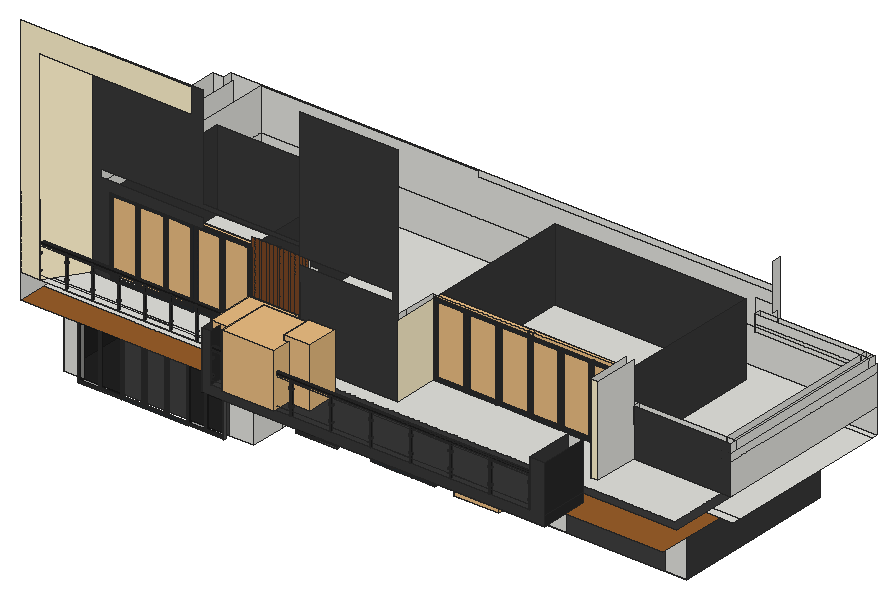
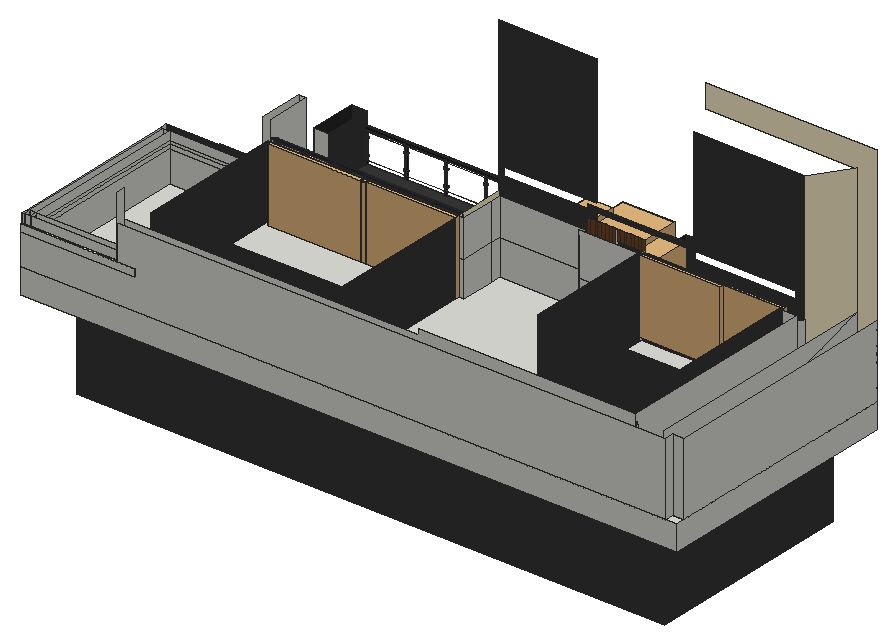
# SketchUp Ruby script. Lengths in inches.
U = 1.inch
M = Sketchup.active_model
def pt(a) = Geom::Point3d.new(a.map { |v| v * U })
def face(e, loops, mat)
  f = e.add_face(loops[0].map { |a| pt(a) })
  loops[1..].each { |l| e.add_face(l.map { |a| pt(a) }).erase! }
  f.material = f.back_material = mat if mat
  f
end
# faces: each face lists its corners as indices into pts; further lists are holes
def faces(e, pts, list, mat = nil) = list.each { |f| face(e, (f[0].is_a?(Array) ? f : [f]).map { |l| l.map { |i| pts[i] } }, mat) }
# xy, xz, yz: faces in a plane at the given z, y or x. An outline is a flat list of corners, or four numbers for a rectangle; further outlines are holes
def ring(l) = l.size == 4 ? [[l[0], l[1]], [l[2], l[1]], [l[2], l[3]], [l[0], l[3]]] : l.each_slice(2).to_a
def flat(e, list, mat, &to3) = list.each { |f| face(e, (f[0].is_a?(Array) ? f : [f]).map { |l| ring(l).map { |u, v| to3.(u, v) } }, mat) }
def xy(e, z, list, mat = nil) = flat(e, list, mat) { |x, y| [x, y, z] }
def xz(e, y, list, mat = nil) = flat(e, list, mat) { |x, z| [x, y, z] }
def yz(e, x, list, mat = nil) = flat(e, list, mat) { |y, z| [x, y, z] }
def lines(e, pts, list) = list.each { |a, b| e.add_line(pt(pts[a]), pt(pts[b])) }
# prism: a flat outline (further loops are holes) pulled along v
def prism(e, loops, v, mat = nil)
  f = face(e, loops, mat); d = Geom::Vector3d.new(v.map { |x| x * U })
  f.pushpull(f.normal.samedirection?(d) ? d.length : -d.length)
end
def box(e, o, s, mat = nil) = prism(e, [[o, [o[0] + s[0], o[1], o[2]], [o[0] + s[0], o[1] + s[1], o[2]], [o[0], o[1] + s[1], o[2]]]], [0, 0, s[2]], mat)
def at(x, y, z, deg = 0) = Geom::Transformation.translation(pt([x, y, z])) * Geom::Transformation.rotation(ORIGIN, Z_AXIS, deg.degrees)
def axes(o, x, y, z) = Geom::Transformation.new([*x, 0, *y, 0, *z, 0, *pt(o).to_a, 1])
def part(name) = M.definitions.add(name)
# library, detail: a bought-in or finely detailed component or shape, given as its bounding box
def library(name, o, s) = part(name).tap { |d| box(d.entities, o, s) }
def detail(e, o, s) = box(e.add_group.entities, o, s)
def put(e, d, t, mat = nil) = e.add_instance(d, t).tap { |i| i.material = mat if mat }
def group(e, t, mat = nil) = e.add_group.tap { |g| g.transformation = t; g.material = mat if mat }.entities
root = M.entities
M.materials.add("Glass_Tinted_Gray").color = [0, 0, 0]
M.materials["Glass_Tinted_Gray"].alpha = 0.125
M.materials.add("Wine2").color = [0, 0, 0]
M.materials["Wine2"].alpha = 0
M.materials.add("[0130_Gainsboro]").color = [39, 45, 50]
M.materials.add("[0131_Silver]").color = [28, 28, 28]
M.materials.add("[0135_DarkGray]").color = [81, 81, 81]
M.materials.add("[Color D01]").color = [255, 242, 204]
M.materials.add("[Color M08]").color = [56, 56, 56]
M.materials.add("[Granite Dark Gray]").color = [40, 40, 40]
M.materials.add("[Mirror 02]").color = [229, 229, 229]
M.materials.add("[Terrazzo Light Blue]").color = [196, 214, 227]
M.materials.add("[Translucent_Glass_Blue]").color = [255, 255, 255]
M.materials["[Translucent_Glass_Blue]"].alpha = 0
M.materials.add("[Wood Floor Dark]").color = [153, 94, 42]
M.materials.add("[Wood Veneer 01]").color = [120, 70, 37]
c1 = part("PENTEK_RP Fineline 50S_Sliding_DoorCase_E1")
box(c1.entities,[0,0,0],[1.51,3.66,99.27],"[0135_DarkGray]")
c2 = part("PENTEK_RP Fineline 50S_SlidingDooe_Case_E2")
box(c2.entities,[0,0,0],[96.25,3.66,1.51],"[0135_DarkGray]")
c3 = part("pentek_RP Fineline 50S_SlidingDoor_Case")
put(c3.entities,c1,at(97.76,0,0))
put(c3.entities,c2,at(1.51,0,0))
put(c3.entities,c1,at(0,0,0))
put(c3.entities,c2,at(1.51,0,97.76))
c4 = part("PENTEK_RP Fineline 50S_SlidingDoor_GlazingBead_2")
box(c4.entities,[0,0,0],[0.56,0.59,94.39],"[0135_DarkGray]")
c5 = part("PENTEK_RP Fineline 50S_SlidingDoor_Glass")
box(c5.entities,[0,0,0],[46.58,0.16,94.39],"Glass_Tinted_Gray")
c6 = part("PENTEK_RP Fineline 50S_SlidingDoor_GlazingBead")
box(c6.entities,[0,0,0],[45.47,0.59,0.56],"[0135_DarkGray]")
c7 = part("PENTEK_RP Fineline 50S_SlidingDoor_Leaf_E1")
xy(c7.entities,0,[[0,0,0.93,1.97],[0.93,1.57,1.49,1.97]],"[0135_DarkGray]")
xy(c7.entities,96.25,[[0,0,0.93,0,0.93,1.57,1.49,1.57,1.49,1.97,0,1.97]],"[0135_DarkGray]")
xz(c7.entities,0,[[0,0,0.93,96.25]],"[0135_DarkGray]")
xz(c7.entities,1.57,[[0.93,0,1.49,95.32],[0.93,95.32,1.49,96.25]],"[0135_DarkGray]")
xz(c7.entities,1.97,[[0,0,1.49,96.25]],"[0135_DarkGray]")
yz(c7.entities,0,[[0,0,1.97,96.25]],"[0135_DarkGray]")
yz(c7.entities,0.93,[[0,0,1.57,0.93],[0,0.93,1.57,95.32],[0,95.32,1.57,96.25]],"[0135_DarkGray]")
yz(c7.entities,1.49,[[1.57,0,1.97,95.32],[1.57,95.32,1.97,96.25]],"[0135_DarkGray]")
c8 = part("PENTEK_RP Fineline 50S_SlidingDoor_Leaf_E2")
xy(c8.entities,0,[[0,0,0,1.57,0.56,1.57,0.56,1.97,46.02,1.97,46.02,1.57,46.58,1.57,46.58,0]],"[0135_DarkGray]")
xy(c8.entities,0.93,[[0,0,46.58,1.57]],"[0135_DarkGray]")
xy(c8.entities,1.49,[[0.56,1.57,46.02,1.97]],"[0135_DarkGray]")
xz(c8.entities,0,[[0,0,46.58,0.93]],"[0135_DarkGray]")
xz(c8.entities,1.57,[[0,0,0.56,0.93],[46.02,0,46.58,0.93],[0.56,0.93,46.02,1.49]],"[0135_DarkGray]")
xz(c8.entities,1.97,[[0.56,0,46.02,1.49]],"[0135_DarkGray]")
yz(c8.entities,0,[[0,0,1.57,0.93]],"[0135_DarkGray]")
yz(c8.entities,0.56,[[1.57,0,1.97,0.93],[1.57,0.93,1.97,1.49]],"[0135_DarkGray]")
yz(c8.entities,46.02,[[1.57,0,1.97,0.93],[1.57,0.93,1.97,1.49]],"[0135_DarkGray]")
yz(c8.entities,46.58,[[0,0,1.57,0.93]],"[0135_DarkGray]")
c9 = part("PENTEK_RP Fineline S_SlidingDoor_Leaf1")
put(c9.entities,c4,at(0.93,0,0.93))
put(c9.entities,c4,at(46.96,0,0.93))
put(c9.entities,c5,at(1.49,1.42,0.93))
put(c9.entities,c6,at(1.49,0,0.93))
put(c9.entities,c5,at(1.49,0.59,0.93),"[Terrazzo Light Blue]")
put(c9.entities,c7,at(0,0,0))
put(c9.entities,c7,axes([48.44,0,0],[-1,0,0],[0,1,0],[0,0,1]))
put(c9.entities,c8,axes([0.93,0,96.25],[1,0,0],[0,1,0],[0,0,-1]))
put(c9.entities,c8,at(0.93,0,0))
put(c9.entities,c6,at(1.49,0,94.77))
c10 = part("PENTEK_RP Fineline 50S_SlidingDoor_Leaf2")
put(c10.entities,c5,at(1.49,1.42,0.93))
put(c10.entities,c6,at(1.49,0,94.77))
put(c10.entities,c4,at(46.96,0,0.93))
put(c10.entities,c5,at(1.49,0.59,0.93),"[Mirror 02]")
put(c10.entities,c4,at(0.93,0,0.93))
put(c10.entities,c7,at(0,0,0))
put(c10.entities,c7,axes([48.44,0,0],[-1,0,0],[0,1,0],[0,0,1]))
put(c10.entities,c6,at(1.49,0,0.93))
put(c10.entities,c8,axes([0.93,0,96.25],[1,0,0],[0,1,0],[0,0,-1]))
put(c10.entities,c8,at(0.93,0,0))
c11 = part("PENTEK - Slimmest Steel Sliding Door / Window\#1")
put(c11.entities,c3,at(0,-1.88,-0.09))
put(c11.entities,c9,at(1.51,-2.27,1.42))
put(c11.entities,c10,at(49.32,-0.3,1.42))
c12 = part("Framed glazing panel")
xy(c12.entities,0,[[0,-0.98,43.07,0],[0,0,43.07,1.4]],"[0130_Gainsboro]")
xy(c12.entities,0.3,[[0.3,-1.43,42.77,-0.98]],"[0130_Gainsboro]")
xy(c12.entities,2.95,[[2.95,-1.43,40.12,-0.63],[2.95,-0.63,40.12,0],[2.95,0,40.12,0.64],[2.95,0.64,40.12,1.4]],"[0130_Gainsboro]")
xy(c12.entities,3.54,[[3.54,-0.63,39.53,0],[3.54,0,39.53,0.64]],"[0130_Gainsboro]")
xy(c12.entities,111.8125,[[3.54,-0.63,39.53,0],[3.54,0,39.53,0.64]],"[0130_Gainsboro]")
xy(c12.entities,112.4,[[2.95,-1.43,40.12,-0.63],[2.95,-0.63,40.12,0],[2.95,0,40.12,0.64],[2.95,0.64,40.12,1.4]],"[0130_Gainsboro]")
xy(c12.entities,115.05,[[0.3,-1.43,42.77,-0.98]],"[0130_Gainsboro]")
xy(c12.entities,115.35,[[0,-0.98,43.07,0],[0,0,43.07,1.4]],"[0130_Gainsboro]")
xz(c12.entities,-1.43,[[[0.3,0.3,42.77,115.05],[2.95,2.95,40.12,112.4]]],"[0130_Gainsboro]")
xz(c12.entities,-0.98,[[[0,0,43.07,115.35],[0.3,0.3,42.77,115.05]]],"[0130_Gainsboro]")
xz(c12.entities,-0.63,[[[2.95,2.95,40.12,112.4],[3.54,3.54,39.53,111.8125]]],"[0130_Gainsboro]")
xz(c12.entities,0,[[3.54,3.54,39.53,111.8125]],"Wine2")
xz(c12.entities,0,[[[0,0,43.07,115.35],[2.95,2.95,40.12,112.4]],[[2.95,2.95,40.12,112.4],[3.54,3.54,39.53,111.8125]]],"[0130_Gainsboro]")
xz(c12.entities,0.64,[[[2.95,2.95,40.12,112.4],[3.54,3.54,39.53,111.8125]]],"[0130_Gainsboro]")
xz(c12.entities,1.4,[[[0,0,43.07,115.35],[2.95,2.95,40.12,112.4]]],"[0130_Gainsboro]")
yz(c12.entities,0,[[-0.98,0,0,115.35],[0,0,1.4,115.35]],"[0130_Gainsboro]")
yz(c12.entities,0.3,[[-1.43,0.3,-0.98,115.05]],"[0130_Gainsboro]")
yz(c12.entities,2.95,[[-1.43,2.95,-0.63,112.4],[-0.63,2.95,0,112.4],[0,2.95,0.64,112.4],[0.64,2.95,1.4,112.4]],"[0130_Gainsboro]")
yz(c12.entities,3.54,[[-0.63,3.54,0,111.8125],[0,3.54,0.64,111.8125]],"[0130_Gainsboro]")
yz(c12.entities,39.53,[[-0.63,3.54,0,111.8125],[0,3.54,0.64,111.8125]],"[0130_Gainsboro]")
yz(c12.entities,40.12,[[-1.43,2.95,-0.63,112.4],[-0.63,2.95,0,112.4],[0,2.95,0.64,112.4],[0.64,2.95,1.4,112.4]],"[0130_Gainsboro]")
yz(c12.entities,42.77,[[-1.43,0.3,-0.98,115.05]],"[0130_Gainsboro]")
yz(c12.entities,43.07,[[-0.98,0,0,115.35],[0,0,1.4,115.35]],"[0130_Gainsboro]")
c13 = part("Glazed screen")
put(c13.entities,c12,axes([90.57,1.43,0],[1.05148,0,0],[0,1,0],[0,0,1]))
put(c13.entities,c12,axes([0,1.43,0],[1.05148,0,0],[0,1,0],[0,0,1]))
put(c13.entities,c12,axes([45.29,1.43,0],[1.05148,0,0],[0,1,0],[0,0,1]))
c14 = library("元件\#5",[-4.39,0,0],[5.37,35.83,90.55])
c15 = library("Group5_1",[-7.56,-66.38,0.11],[6.33,135.04,120.95])
c16 = library("Pot+Plant",[-20.81,-17.08,-0.03],[39.86,39.43,41.33])
c17 = library("Potted broadleaf plant",[-29.7,0,-10.87],[31.67,38.52,72.45])
c18 = library("Plant+++Pot",[-21.48,-119.36,-205.6875],[86.44,86.43,89.41])
c19 = part("Monstera_Pot_Quarter")
detail(c19.entities,[0.23,0.23,0],[9.32,9.32,13.9])
c20 = part("Monstera_Stem")
p = [[0.53,2.46,1.55],[0.55,2.41,0.71],[0.58,2.34,0.01],[0.58,2.59,0.01],[0.53,2.71,1.56],[0.48,2.66,3.11],
  [0.43,2.45,4.65],[0.38,2.07,6.15],[0.34,1.53,7.61],[0.29,0.84,9],[0.25,0,10.3125],[0.27,0.15,9.7],
  [0.3,0.62,8.89],[0.3,0.62,8.88],[0.34,1.3,7.51],[0.38,1.83,6.08],[0.43,2.2,4.6],[0.48,2.41,3.09],
  [0.53,2.46,1.5625],[0.33,2.59,0],[0.28,2.71,1.55],[0.23,2.66,3.1],[0.18,2.45,4.64],[0.13,2.07,6.15],
  [0.09,1.53,7.6],[0.04,0.84,8.99],[0,0,10.3]]
faces(c20.entities,p,[[0,1,2,3,4,5,6,7,8,9,10,11,12,13,14,15,16,17,18],[19,20,4,3],[20,21,5,4],[21,22,6,5],[22,23,7,6],[23,24,8,7],[24,25,9,8],[25,26,10,9]])
c21 = part("Monstera_Leaf_Half")
xy(c21.entities,0,[[9.39,-0.71,9.39,17.36,8.6,18.11,7.67,18.6875,6.64,19.0625,5.75,18.99,4.86,18.84,4,18.6,3.16,18.29,2.35,17.9,1.58,17.4375,0.86,16.91,0.33,15.95,0,14.91,0.64,15.5625,1.37,16.12,2.17,16.57,3.02,16.9,3.92,17.11,4.83,17.19,5.74,17.15,5.1,16.89,4.48,16.59,3.87,16.25,3.28,15.88,2.72,15.48,2.18,15.04,1.67,14.57,1.29,14.3,0.95,13.98,0.65,13.62,0.4,13.22,0.21,12.79,0.08,12.34,0.01,11.88,0.16,11.13,0.36,10.5,1.02,11.46,1.77,12.35,2.62,13.16,3.55,13.87,4.55,14.48,5.6,14.98,6.7,15.37,5.51,14.66,4.41,13.82,3.42,12.85,2.56,11.76,1.84,10.57,1.27,9.31,1.03,8.54,1.39,7.56,1.75,8.34,2.22,9.05,2.79,9.68,3.45,10.22,4.19,10.65,4.99,10.95,5.82,11.14,5.92,10.73,4.92,9.82,4.09,8.76,3.45,7.57,3.03,6.3,2.89,5.38,3.67,4.53,4.23,5.52,5,6.36,5.95,6.99,7.01,7.39,8.14,7.54,7.33,6.92,6.62,6.2,6,5.39,5.8125,4.66,5.76,3.92,5.83,3.17,6.03,2.45,7.95,4.19,6.73,2.06,6.96,1.71,7.24,1.375,7.55,1.08,7.89,0.8125,8.25,0.59,8.47,0.46,8.67,0.3125,8.86,0.14,9.03,-0.05,9.17,-0.26,9.29,-0.48]])
c22 = part("Monstera_Leaf_Half2")
xy(c22.entities,0,[[0,0,0.0625,0.14,0.14,0.28,0.23,0.41,0.33,0.53,0.44,0.64,0.57,0.73,0.7,0.8125,1.02,1.05,1.3125,1.33,1.58,1.63,0.92,3.26,1.66,1.76,1.8,1.96,2,2.31,1.99,2.65,1.9375,2.97,1.85,3.29,1.72,3.6,1.55,3.88,1.35,4.15,1.11,4.38,1.45,4.3,1.78,4.18,2.09,4.02,2.38,3.82,2.65,3.6,2.88,3.34,3.09,3.05,3.42,3.43,3.31,3.8125,3.15,4.18,2.96,4.54,2.74,4.87,2.48,5.18,2.19,5.46,1.88,5.7,1.88,6.2,2.29,6.15,2.68,6.02,3.05,5.83,3.38,5.58,3.67,5.27,3.89,4.93,4.06,4.54,4.28,4.99,4.17,5.67,3.98,6.32,3.7,6.94,3.34,7.52,2.9,8.04,2.4,8.51,2.18,8.66,2.18,8.85,2.46,8.8,3.05,8.58,3.57,8.25,4.02,7.82,4.37,7.3,4.61,6.73,4.72,6.12,5.05,6.79,4.86,7.39,4.6,7.96,4.26,8.49,3.85,8.97,3.39,9.4,2.87,9.75,2.3125,10.04,2.93,10.08,3.55,9.98,4.13,9.77,4.66,9.44,5.11,9,5.46,8.49,5.7,7.92,5.7,8.79,5.36,9.78,4.75,10.625,3.92,11.25,2.9375,11.6,1.9,11.65,0.89,11.39,0,10.84]])
c23 = part("Monstera_Leaf")
put(c23.entities,c21,axes([0,0.43,2.5],[0.6,0,0],[0,0.6,0],[0,0,1]))
put(c23.entities,c22,axes([5.63,0,2.5],[0.89879,0,-0.43837],[0,1,0],[0.43837,0,0.89879]))
c24 = part("Plant_Potted_Monstera")
g1 = group(c24.entities,at(-31.76,-2.48,0))
put(g1,c19,axes([41.19,13.38,0],[-1.05801,1.45623,0],[-1.45623,-1.05801,0],[0,0,1.8]))
put(g1,c19,axes([-4.47,6.15,0],[1.7119,-0.55623,0],[0.55623,1.7119,0],[0,0,1.8]))
put(g1,c19,axes([0,34.37,0],[0,-1.8,0],[1.8,0,0],[0,0,1.8]))
put(g1,c19,axes([28.22,38.84,0],[-1.7119,-0.55623,0],[0.55623,-1.7119,0],[0,0,1.8]))
put(g1,c19,axes([20.99,-6.82,0],[1.05801,1.45623,0],[-1.45623,1.05801,0],[0,0,1.8]))
g2 = group(c24.entities,at(-45.35,-10.84,22.35))
put(g2,c20,axes([31.57,11.47,0.05],[2.4,0,0],[0,2.4,0],[0,0,2.4]))
put(g2,c20,axes([37.07,37.75,-0.89],[-1.58858,0.45043,0.25253],[-0.40158,-1.59114,0.31185],[0.32464,0.23586,1.62148]))
put(g2,c20,axes([35.38,18.48,0],[3.25902,1.8816,0],[-2.0384,3.53061,0],[0,0,5.08031]))
put(g2,c20,axes([43.34,34.52,0.05],[-2.22411,3.85227,0],[-3.85227,-2.22411,0],[0,0,3.86995]))
put(g2,c20,axes([25.97,39.07,0.05],[-3.61063,-0.96747,0],[0.96747,-3.61063,0],[0,0,3.738]))
put(g2,c20,axes([21.76,18.96,0.05],[3.25939,-2.64884,0],[2.64884,3.25939,0],[0,0,4.2]))
put(g2,c20,axes([46.1,26.35,-0.74],[-0.50009,2.70618,0.3788],[-2.67394,-0.57497,0.46778],[0.59215,-0.31088,2.43223]))
put(g2,c20,axes([20.02,34.71,0.05],[-1.28976,-1.28976,0],[1.28976,-1.28976,0],[0,0,1.824]))
put(g2,c20,axes([15.69,19.9375,-0.89],[1.34133,-2.40299,0.42089],[2.34844,1.40191,0.51975],[-0.66056,0.10462,2.70247]))
put(g2,c23,axes([-0.47,22.84,6.14],[1.06874,-1.68333,0.43106],[0.69416,0.81107,1.44626],[-1.54881,-0.6934,1.13225]))
put(g2,c23,axes([50.87,17.94,4.27],[0.87503,1.76297,0.48288],[-0.72296,-0.14022,1.47584],[1.65009,-1.01401,0.5767]))
put(g2,c23,axes([49.79,39.97,-5.14],[-1.19278,1.56557,0.53653],[-0.62569,-0.953,1.38984],[1.49489,0.73546,1.17729]))
put(g2,c23,axes([50.65,23.15,27.2],[-0.38969,1.51702,-0.48773],[-0.81041,0.17386,1.24069],[1.35916,0.56845,0.81291]))
put(g2,c23,axes([26.42,52.09,4.7],[-1.67848,-1.12654,-0.48514],[0.50255,-1.2731,1.21752],[-1.0859,0.98249,1.47556]))
put(g2,c22,axes([32.94,54.6,23.93],[-1.59866,-0.5353,-1.42606],[-0.72066,-1.45568,1.3543],[-1.26669,1.65244,1.1021]))
put(g2,c21,axes([43.86,52.61,29.01],[-1.19529,0.14595,-0.47916],[-0.43239,-0.87341,0.81258],[-0.43769,1.71986,1.6157]))
put(g2,c22,axes([12.98,3.28,29],[2.16876,-0.96374,-0.35734],[0.84721,1.41614,1.32259],[-0.36343,-1.49947,1.83834]))
put(g2,c21,axes([3.26,12.46,26.83],[1.07397,-0.91411,0.29082],[0.50833,0.84969,0.79355],[-1.27737,-0.92524,1.80894]))
put(g2,c21,axes([30.81,4.39,33.875],[1.04828,0.47771,0],[-0.26309,0.57732,1.05032],[0.8619,-1.89133,1.14696]))
put(g2,c22,axes([40.84,8.47,33.13],[1.19248,1.54471,-0.50279],[-0.43849,0.96221,1.75054],[1.54056,-1.35089,1.03088]))
put(g2,c23,axes([26.17,-0.34,3.65],[1.93185,0,0.51764],[-0.36603,1.41421,1.36603],[-0.36603,-1.41421,1.36603]))
c25 = part("Group\#11")
xy(c25.entities,0,[[0,0,0.39,2.125]],"[0131_Silver]")
xy(c25.entities,1.5,[[0,0,0.39,2.125]],"[0131_Silver]")
xz(c25.entities,0,[[0,0,0.39,1.5]],"[0131_Silver]")
xz(c25.entities,2.125,[[0,0,0.39,1.5]],"[0131_Silver]")
yz(c25.entities,0,[[0,0,2.125,1.5]],"[0131_Silver]")
yz(c25.entities,0.39,[[0,0,2.125,1.5]],"[0131_Silver]")
c26 = part("Glass railing panel")
xy(c26.entities,0,[[-0.59,0,0,63.98]])
xy(c26.entities,37.71,[[-0.59,0,0,63.98]])
xz(c26.entities,0,[[-0.59,0,0,37.71]])
xz(c26.entities,63.98,[[-0.59,0,0,37.71]])
yz(c26.entities,-0.59,[[0,0,63.98,37.71]])
yz(c26.entities,0,[[0,0,63.98,0,63.98,37.71,0,37.71,0,30.53,1.75,30.53,1.75,28.71,0,28.71],[-0.4,28.71,0,30.53],[0,28.71,1.75,30.53]])
p = [[0,63.98,30.53],[0.39,63.98,30.53]]
lines(c26.entities,p,[[0,1]])
put(c26.entities,c25,axes([0,62.22,28.71],[1,0,0],[0,1.01246,0],[0,0,1.2158]))
put(c26.entities,c25,axes([0,62.22,6.27],[1,0,0],[0,1.01246,0],[0,0,1.2158]))
put(c26.entities,c25,axes([0,0.6,28.71],[1,0,0],[0,1.01246,0],[0,0,1.2158]))
put(c26.entities,c25,axes([0,0.6,6.27],[1,0,0],[0,1.01246,0],[0,0,1.2158]))
put(c26.entities,c25,axes([-0.98,0.6,28.71],[1,0,0],[0,1.01246,0],[0,0,1.2158]))
put(c26.entities,c25,axes([-0.98,62.22,6.27],[1,0,0],[0,1.01246,0],[0,0,1.2158]))
put(c26.entities,c25,axes([-0.98,0.6,6.27],[1,0,0],[0,1.01246,0],[0,0,1.2158]))
put(c26.entities,c25,axes([-0.98,62.22,28.71],[1,0,0],[0,1.01246,0],[0,0,1.2158]))
c27 = part("Group\#1")
xz(c27.entities,0,[[0,0,1.97,38.58]])
xz(c27.entities,1.97,[[0,0,1.97,38.58]])
yz(c27.entities,0,[[0,0,1.97,37.71]])
yz(c27.entities,1.97,[[0,0,1.97,37.71]])
c28 = part("Glass railing")
xy(c28.entities,37.71,[[2.51,0,3.15,0.39,3.15,0]])
xy(c28.entities,37.71,[[0,0,0.54,520.67],[2.51,0,2.51,63.58,3.15,0.39],[3.15,0.39,2.51,63.58,2.51,520.67,3.15,520.67]],"[0131_Silver]")
xy(c28.entities,38.58,[[0.54,496.0625,2.51,520.67]])
xy(c28.entities,38.58,[[0.54,0,2.51,496.0625]],"[0131_Silver]")
xy(c28.entities,40.46,[[0,0,3.15,520.67]],"[0131_Silver]")
xz(c28.entities,0,[[0,37.71,0.54,37.71,0.54,38.58,2.51,38.58,2.51,37.71,3.15,37.71,3.15,40.46,0,40.46]],"[0131_Silver]")
xz(c28.entities,520.67,[[0,37.71,0,40.46,3.15,40.46,3.15,37.71,2.51,37.71,2.51,38.58,0.54,38.58,0.54,37.71]])
yz(c28.entities,0,[[0,37.71,520.67,40.46]],"[0131_Silver]")
yz(c28.entities,0.54,[[496.0625,37.71,520.67,38.58]])
yz(c28.entities,0.54,[[0,37.71,496.0625,38.58]],"[0131_Silver]")
yz(c28.entities,2.51,[[0,37.71,496.0625,38.58],[496.0625,37.71,520.67,38.58]])
yz(c28.entities,3.15,[[0,37.71,520.67,40.46]],"[0131_Silver]")
put(c28.entities,c26,axes([1.8,65.35,3.9375],[1,0,0],[0,0.98769,0],[0,0,0.8225]),"[Translucent_Glass_Blue]")
put(c28.entities,c26,axes([1.8,130.31,3.9375],[1,0,0],[0,0.98769,0],[0,0,0.8225]),"[Translucent_Glass_Blue]")
put(c28.entities,c26,axes([1.8,195.28,3.9375],[1,0,0],[0,0.98769,0],[0,0,0.8225]),"[Translucent_Glass_Blue]")
put(c28.entities,c26,axes([1.8,260.24,3.9375],[1,0,0],[0,0.98769,0],[0,0,0.8225]),"[Translucent_Glass_Blue]")
put(c28.entities,c26,axes([1.8,325.2,3.9375],[1,0,0],[0,0.98769,0],[0,0,0.8225]),"[Translucent_Glass_Blue]")
put(c28.entities,c26,axes([1.8,390.16,3.9375],[1,0,0],[0,0.98769,0],[0,0,0.8225]),"[Translucent_Glass_Blue]")
put(c28.entities,c26,axes([1.8,455.12,3.9375],[1,0,0],[0,0.98769,0],[0,0,0.8225]),"[Translucent_Glass_Blue]")
put(c28.entities,c26,axes([1.8,0.39,3.9375],[1,0,0],[0,0.98769,0],[0,0,0.8225]),"[Translucent_Glass_Blue]")
put(c28.entities,c27,at(0.54,128.9375,0),"[0131_Silver]")
g3 = group(c28.entities,at(0.54,63.98,0),"[0131_Silver]")
xz(g3,0,[[0,0,1.97,38.58]])
xz(g3,1.97,[[0,0,1.97,38.58]])
yz(g3,0,[[0,0,1.97,37.71]])
yz(g3,1.97,[[0,0,1.97,37.71]])
put(c28.entities,c27,at(0.54,193.9,0),"[0131_Silver]")
put(c28.entities,c27,at(0.54,258.86,0),"[0131_Silver]")
put(c28.entities,c27,at(0.54,323.82,0),"[0131_Silver]")
put(c28.entities,c27,at(0.54,388.78,0),"[0131_Silver]")
put(c28.entities,c27,at(0.54,453.74,0),"[0131_Silver]")
put(c28.entities,c27,at(0.54,518.7,0),"[0131_Silver]")
c29 = part("Glass+Railing (1)")
put(c29.entities,c28,axes([0,0,0],[1,0,0],[0,0.95652,0],[0,0,1]),"[0131_Silver]")
xy(root,52.0625,[[231.01,347.22,543.63,347.22,543.63,420.5625,1199.95,420.5625,1199.95,570.63,416.44,570.63,416.44,556.88,399.26,556.88,399.26,497.29,231.01,497.29],[231.01,497.29,399.26,497.29,399.26,556.88,416.44,556.88,416.44,570.63,1199.95,570.63,1199.95,693.77,231.01,693.77]],"[Color M08]")
xy(root,168.9375,[[263.51,336.9375,504.95,347.22]])
xy(root,172.0625,[[204.29,336.9375,549.32,336.9375,549.32,406.8125,566.51,406.8125,566.51,420.5625,543.63,420.5625,543.63,347.22,231.01,347.22,231.01,693.77,1286.86,693.77,1286.86,701.99,204.29,701.99],[633.8,406.8125,687.15,420.5625],[797.18,406.8125,828.83,420.5625],[903,406.8125,999.61,420.5625],[999.61,406.8125,1165.59,420.5625],
  [1165.59,406.8125,1286.86,420.5625],[1199.95,420.5625,1286.86,693.77]])
xy(root,172.0625,[[[204.29,290.49,204.29,336.9375,549.32,336.9375,549.32,406.8125,566.51,406.8125,566.51,420.5625,543.63,420.5625,543.63,347.22,231.01,347.22,231.01,693.77,1199.95,693.77,1199.95,420.5625,903,420.5625,903,406.8125,1264.2,406.8125,1264.2,290.49],[971.33,360.8,979.08,373.34],[971.33,338.36,979.08,350.9],[971.33,316.67,979.08,329.21],[971.33,295.36,979.08,307.9]]],"[Wood Floor Dark]")
xy(root,198,[[566.56,212.24,1115.11,290.49],[1115.11,212.24,1132.55,290.49]],"[Granite Dark Gray]")
xy(root,213.5625,[[204.29,290.49,236.62,687.48],[236.62,290.49,236.62,687.48,282.79,687.48,282.79,356.52,276.18,347.0625,246.76,305],[236.62,290.49,566.56,290.49,566.56,305,246.76,305],[566.56,290.49,581.07,305],[246.76,305,1272.34,305,1272.34,401,1126.93,401,1126.93,328.1875,1115.11,328.1875,1115.11,401,1108.3,401,1108.3,411.84,1110.75,411.84,1110.75,652.46,796.43,652.46,796.43,328.1875,634.74,328.1875,634.74,347.0625,540.88,347.0625,540.88,566.77,307.88,566.77,307.88,347.0625,276.18,347.0625],
  [634.74,328.1875,634.74,347.0625,540.88,347.0625,540.88,356.52,641.68,356.52,641.68,338.65,787.31,338.65,787.31,411.84,796.43,411.84,796.43,328.1875],[641.68,338.65,787.31,338.65,787.31,411.84,796.43,411.84,796.43,652.46,1110.75,652.46,1110.75,411.84,1272.34,411.84,1272.34,687.48,282.79,687.48,282.79,356.52,307.88,356.52,307.88,566.77,540.88,566.77,540.88,356.52,641.68,356.52],[276.18,347.0625,282.79,356.52,307.88,356.52,307.88,347.0625],[1108.3,401,1108.3,411.84,1272.34,411.84,1272.34,687.48,222.11,687.48,222.11,701.99,1286.86,701.99,1286.86,401],[204.29,687.48,222.11,701.99]])
xy(root,213.5625,[[581.07,212.24,1107.49,212.24,1107.49,290.49,1286.86,290.49,1286.86,401,1272.34,401,1272.34,305,581.07,305]],"[Color M08]")
xy(root,276.9375,[[1272.34,411.84,1283.18,687.48],[1283.18,411.84,1286.86,687.48],[1098.24,687.48,1272.34,698.3125],[1272.34,687.48,1283.18,698.3125],[1283.18,687.48,1286.86,698.3125],
  [1098.24,698.3125,1127.04,701.99],[1127.04,698.3125,1286.86,701.99]])
xz(root,212.24,[[566.56,198,1132.55,198,1132.55,291.625,1107.49,291.625,1107.49,213.5625,581.07,213.5625,581.07,293.375,566.56,293.375]],"[Color M08]")
xz(root,290.49,[[1115.11,198,1132.55,213.5625],[1107.49,213.5625,1132.55,291.625]])
xz(root,290.49,[[204.29,213.5625,236.62,213.5625,236.62,546.625,485.87,546.625,485.87,585.5,204.29,585.5]],"[Color D01]")
xz(root,305,[[566.56,213.5625,581.07,293.375]])
xz(root,328.1875,[[1115.11,213.5625,1126.93,359.12]],"[Color D01]")
xz(root,328.1875,[[634.74,213.5625,796.43,213.5625,796.43,585.5,634.74,585.5,634.74,372.12,787.93,372.12,787.93,359.31,634.74,359.31]],"[Color M08]")
xz(root,338.65,[[641.68,213.5625,787.31,271.9375],[641.68,271.9375,787.31,333.5625]])
xz(root,347.0625,[[634.74,213.5625,635.75,359.31]])
xz(root,347.0625,[[276.18,213.5625,307.88,213.5625,307.88,342.3125,460.53,342.3125,460.53,359.31,291.49,359.31,291.49,372.12,634.74,372.12,634.74,378.9375,460.02,378.9375,460.02,547.25,276.18,547.25]],"[Color M08]")
xz(root,347.0625,[[540.88,213.5625,545.75,359.31],[545.75,213.5625,551.75,359.31],[551.75,213.5625,557.75,359.31],[557.75,213.5625,563.75,359.31],[563.75,213.5625,569.75,359.31],
  [569.75,213.5625,575.75,359.31],[575.75,213.5625,581.75,359.31],[581.75,213.5625,587.75,359.31],[587.75,213.5625,593.75,359.31],[593.75,213.5625,599.75,359.31],
  [599.75,213.5625,605.75,359.31],[605.75,213.5625,611.75,359.31],[611.75,213.5625,617.75,359.31],[617.75,213.5625,623.75,359.31],[623.75,213.5625,629.75,359.31],
  [629.75,213.5625,634.74,359.31]],"[Wood Veneer 01]")
xz(root,347.22,[[231.01,52.0625,231.01,172.0625,543.63,172.0625,543.63,52.0625,504.95,52.0625,504.95,168.9375,263.51,168.9375,263.51,52.0625]])
xz(root,348.35,[[582.33,213.5625,587.2,213.5625,587.2,359.31,585.33,359.31,585.33,342.3125,582.33,342.3125]])
xz(root,356.52,[[282.79,213.5625,307.88,271.9375],[540.88,213.5625,641.68,271.9375],[282.79,271.9375,307.88,342.3125],[540.88,271.9375,641.68,342.3125]])
xz(root,401,[[1115.11,213.5625,1126.93,264.6875],[1115.11,264.6875,1126.93,276.9375],[1115.11,276.9375,1126.93,291.625],[1126.93,276.9375,1127.04,291.625]])
xz(root,401,[[1126.93,213.5625,1286.86,213.5625,1286.86,291.625,1127.04,291.625,1127.04,264.6875,1126.93,264.6875]],"[Color M08]")
xz(root,401,[[1108.3,213.5625,1115.11,333.5625]],"[Granite Dark Gray]")
xz(root,411.84,[[787.31,213.5625,796.43,271.9375],[1108.3,213.5625,1110.75,271.9375],[1110.75,213.5625,1116.92,271.9375],[1116.92,213.5625,1272.34,213.5625,1272.34,264.6875,1127.04,264.6875,1127.04,271.9375,1116.92,271.9375],[1127.04,264.6875,1272.34,271.9375],
  [787.31,271.9375,796.43,333.5625],[1108.3,271.9375,1110.75,291.625],[1110.75,271.9375,1116.92,291.625],[1116.92,271.9375,1127.04,291.625],[1127.04,271.9375,1272.34,276.9375],
  [1127.04,276.9375,1272.34,291.625],[1272.34,276.9375,1283.18,291.625],[1283.18,276.9375,1286.86,291.625]])
xz(root,420.5625,[[543.63,52.0625,566.51,172.0625],[633.8,52.0625,687.15,172.0625],[797.18,52.0625,828.83,172.0625],[903,52.0625,999.61,172.0625],[1165.59,52.0625,1199.95,172.0625]])
xz(root,566.77,[[307.88,213.5625,540.88,345.5]],"[Color M08]")
xz(root,652.46,[[796.43,213.5625,1110.75,333.5625]],"[Color M08]")
xz(root,687.48,[[204.29,213.5625,222.11,333.5625],[236.62,213.5625,282.79,213.5625,282.79,333.5625],[282.79,213.5625,1272.34,213.5625,1272.34,264.6875,1098.24,264.6875,1098.24,271.9375,282.79,271.9375],[1098.24,264.6875,1272.34,271.9375],[282.79,271.9375,1098.24,271.9375,1098.24,316.5625,1127.04,316.5625,1127.04,333.5625,641.68,333.5625,641.68,342.3125,282.79,342.3125],
  [1098.24,271.9375,1272.34,276.9375],[1098.24,276.9375,1272.34,291.625],[1272.34,276.9375,1283.18,291.625],[1283.18,276.9375,1286.86,291.625]])
xz(root,693.77,[[231.01,52.0625,1199.95,172.0625]],"[Color M08]")
xz(root,698.3125,[[1098.24,276.9375,1127.04,291.625],[1127.04,276.9375,1272.34,291.625],[1272.34,276.9375,1283.18,291.625],[1283.18,276.9375,1286.86,291.625]])
xz(root,701.99,[[204.29,172.0625,1286.86,213.5625],[222.11,213.5625,222.11,333.5625,1127.04,333.5625,1127.04,276.9375,1098.24,276.9375,1098.24,264.6875,1286.86,264.6875,1286.86,213.5625],[1098.24,264.6875,1286.86,276.9375]])
yz(root,204.29,[[290.49,172.0625,701.99,213.5625],[290.49,213.5625,687.48,333.5625]])
yz(root,222.11,[[687.48,213.5625,701.99,333.5625]])
yz(root,231.01,[[347.22,52.0625,693.77,172.0625]],"[Color M08]")
yz(root,236.62,[[290.49,213.5625,687.48,213.5625,290.49,333.5625],[687.48,213.5625,687.48,333.5625,290.49,333.5625]])
yz(root,282.79,[[356.52,213.5625,687.48,271.9375],[356.52,271.9375,687.48,342.3125]])
yz(root,307.88,[[347.0625,213.5625,356.52,342.3125]])
yz(root,307.88,[[356.52,213.5625,566.77,345.5]],"[Color M08]")
yz(root,540.88,[[347.0625,213.5625,356.52,342.3125]])
yz(root,540.88,[[356.52,213.5625,566.77,271.9375],[356.52,271.9375,566.77,345.5]],"[Color M08]")
yz(root,543.63,[[347.22,52.0625,406.8125,172.0625],[406.8125,52.0625,420.5625,172.0625]])
yz(root,566.56,[[212.24,198,290.49,213.5625],[212.24,213.5625,290.49,293.375]],"[Color M08]")
yz(root,566.56,[[290.49,213.5625,305,293.375]],"[Granite Dark Gray]")
yz(root,581.07,[[212.24,213.5625,305,293.375]],"[Granite Dark Gray]")
yz(root,634.74,[[328.1875,213.5625,347.0625,333.5625]],"[Granite Dark Gray]")
yz(root,641.68,[[338.65,213.5625,356.52,271.9375],[338.65,271.9375,356.52,333.5625]])
yz(root,787.31,[[338.65,213.5625,356.52,271.9375],[356.52,213.5625,411.84,271.9375],[338.65,271.9375,356.52,333.5625],[356.52,271.9375,411.84,333.5625]])
yz(root,796.43,[[328.1875,213.5625,411.84,333.5625]],"[Color D01]")
yz(root,796.43,[[411.84,213.5625,652.46,333.5625]],"[Color M08]")
yz(root,1098.24,[[687.48,264.6875,701.99,276.9375],[687.48,276.9375,698.3125,291.625]])
yz(root,1107.49,[[212.24,213.5625,290.49,291.625]],"[Color M08]")
yz(root,1108.3,[[401,213.5625,411.84,333.5625]])
yz(root,1110.75,[[411.84,213.5625,652.46,333.5625]],"[Color M08]")
yz(root,1115.11,[[328.1875,213.5625,401,359.12]])
yz(root,1126.93,[[328.1875,213.5625,401,359.12]])
yz(root,1127.04,[[401,264.6875,411.84,276.9375],[401,276.9375,411.84,291.625],[698.3125,276.9375,701.99,276.9375,701.99,378.9375,687.48,378.9375,687.48,302.375,698.3125,302.375]])
yz(root,1132.55,[[212.24,198,290.49,213.5625],[212.24,213.5625,290.49,291.625]],"[Granite Dark Gray]")
yz(root,1199.95,[[420.5625,52.0625,693.77,172.0625]],"[Color M08]")
yz(root,1272.34,[[411.84,213.5625,687.48,264.6875],[411.84,264.6875,687.48,271.9375],[411.84,271.9375,687.48,276.9375],[411.84,276.9375,687.48,291.625],[687.48,276.9375,698.3125,291.625]])
yz(root,1283.18,[[411.84,276.9375,687.48,291.625],[687.48,276.9375,698.3125,291.625]])
yz(root,1286.86,[[401,213.5625,701.99,264.6875],[401,264.6875,701.99,276.9375],[401,276.9375,411.84,291.625],[411.84,276.9375,687.48,291.625],[687.48,276.9375,698.3125,291.625]])
p = [[236.62,290.49,213.5625],[246.76,305,213.5625],[276.18,347.0625,213.5625],[276.18,347.0625,333.5625],[276.18,347.0625,547.25],[236.62,290.49,547.25],
  [236.62,290.49,546.625],[236.62,290.49,333.5625],[282.79,356.52,213.5625],[282.79,356.52,333.5625],[282.79,356.52,271.9375],[1272.34,411.84,264.6875],
  [1272.34,401,264.6875],[1272.34,411.84,276.9375],[1272.34,401,276.9375],[1283.18,411.84,276.9375],[1283.18,401,276.9375]]
faces(root,p,[[0,1,2,3,4,5,6,7]],"[Color D01]")
faces(root,p,[[8,2,3,9,10]])
lines(root,p,[[11,12],[13,14],[15,16]])
put(root,c11,axes([263.51,336.9375,52.08],[0.73,0,0],[0,1,0],[0,0,1.18]))
put(root,c11,axes([443.28,336.9375,52.08],[0.6132,0,0],[0,1,0],[0,0,1.18]))
put(root,c13,axes([334.88,335.06,52.0625],[0.81654,0,0],[0,1,0],[0,0,1.0073]))
put(root,c13,axes([687.89,408.21,52.0625],[0.78162,0,0],[0,1,0],[0,0,1.04027]))
put(root,c11,axes([565.01,409.08,52.18],[0.69298,0,0],[0,1,0],[0,0,1.23782]),"[Color M08]")
put(root,c14,axes([828.83,405.78,52.53],[0,-1.32,0],[2.07007,0,0],[0,0,1.32]))
put(root,c15,axes([873.43,410.61,212.5],[0,-1,0],[1.16,0,0],[0,0,1]))
put(root,c15,axes([1024.07,410.61,212.5],[0,-1,0],[1.2,0,0],[0,0,1]))
put(root,c16,axes([607.74,265.99,213.6],[2,0,0],[0,2,0],[0,0,2]))
put(root,c17,axes([719.81,238.8125,228.13],[1.34,0,0],[0,1.34,0],[0,0,1.34]))
put(root,c13,axes([307.88,347.0625,213.5625],[1,0,0],[0,1,0],[0,0,1.11613]))
put(root,c13,axes([443.74,349.89,213.5625],[1,0,0],[0,1,0],[0,0,1.11613]))
put(root,c18,at(623.2,328.1875,419.25))
put(root,c24,at(674.8125,244,213.5625))
put(root,c13,axes([796.43,401.34,213.5625],[1.18427,0,0],[0,1,0],[0,0,1.04867]))
put(root,c13,axes([956.97,399.94,213.5625],[1.11,0,0],[0,1,0],[0,0,1.04867]))
put(root,c29,axes([581.07,215.39,213.5625],[0,-1,0],[1.05701,0,0],[0,0,1.41]))
put(root,c29,axes([236.62,293.64,213.5625],[0,-1,0],[0.69162,0,0],[0,0,1.41]))
put(root,c15,at(472.22,352.77,221.25,-90))
put(root,c15,at(372.47,345.84,221.25,-90))
